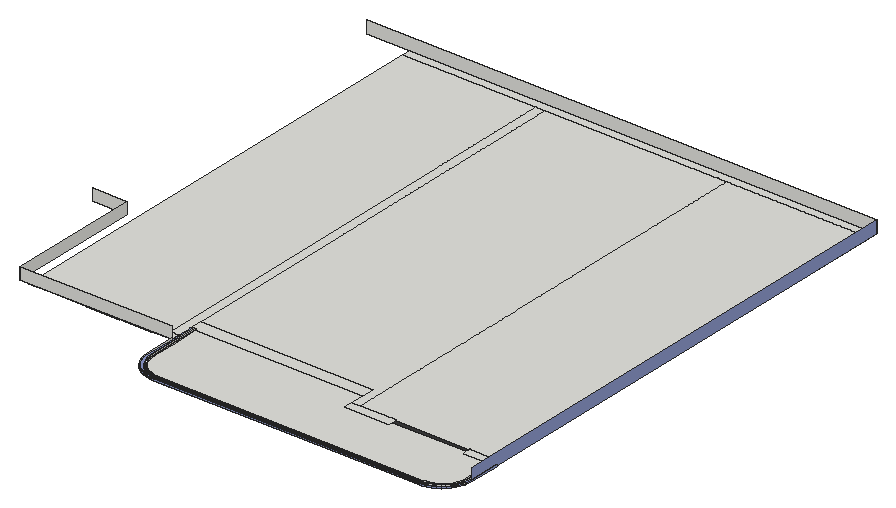
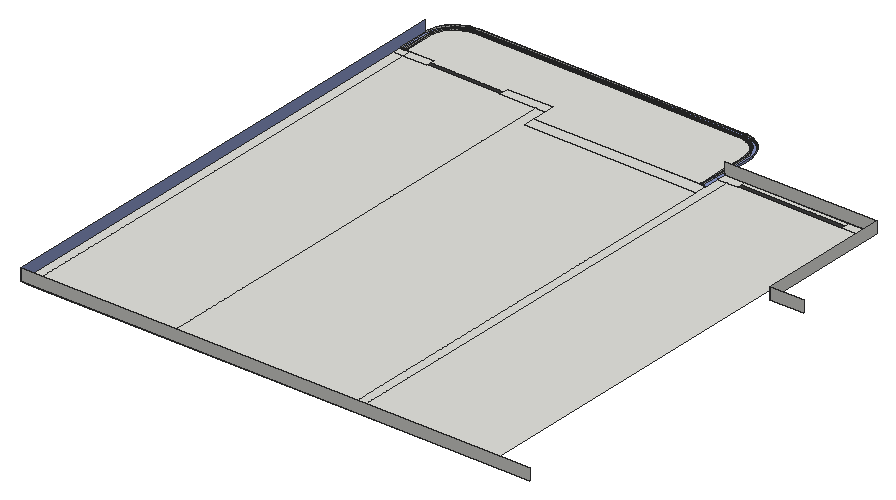
# SketchUp Ruby script. Lengths in inches.
U = 1.inch
M = Sketchup.active_model
def pt(a) = Geom::Point3d.new(a.map { |v| v * U })
def face(e, loops, mat)
  f = e.add_face(loops[0].map { |a| pt(a) })
  loops[1..].each { |l| e.add_face(l.map { |a| pt(a) }).erase! }
  f.material = f.back_material = mat if mat
  f
end
# faces: each face lists its corners as indices into pts; further lists are holes
def faces(e, pts, list, mat = nil) = list.each { |f| face(e, (f[0].is_a?(Array) ? f : [f]).map { |l| l.map { |i| pts[i] } }, mat) }
# xy, xz, yz: faces in a plane at the given z, y or x. An outline is a flat list of corners, or four numbers for a rectangle; further outlines are holes
def ring(l) = l.size == 4 ? [[l[0], l[1]], [l[2], l[1]], [l[2], l[3]], [l[0], l[3]]] : l.each_slice(2).to_a
def flat(e, list, mat, &to3) = list.each { |f| face(e, (f[0].is_a?(Array) ? f : [f]).map { |l| ring(l).map { |u, v| to3.(u, v) } }, mat) }
def xy(e, z, list, mat = nil) = flat(e, list, mat) { |x, y| [x, y, z] }
def xz(e, y, list, mat = nil) = flat(e, list, mat) { |x, z| [x, y, z] }
def yz(e, x, list, mat = nil) = flat(e, list, mat) { |y, z| [x, y, z] }
def lines(e, pts, list) = list.each { |a, b| e.add_line(pt(pts[a]), pt(pts[b])) }
# prism: a flat outline (further loops are holes) pulled along v
def prism(e, loops, v, mat = nil)
  f = face(e, loops, mat); d = Geom::Vector3d.new(v.map { |x| x * U })
  f.pushpull(f.normal.samedirection?(d) ? d.length : -d.length)
end
def box(e, o, s, mat = nil) = prism(e, [[o, [o[0] + s[0], o[1], o[2]], [o[0] + s[0], o[1] + s[1], o[2]], [o[0], o[1] + s[1], o[2]]]], [0, 0, s[2]], mat)
def at(x, y, z, deg = 0) = Geom::Transformation.translation(pt([x, y, z])) * Geom::Transformation.rotation(ORIGIN, Z_AXIS, deg.degrees)
def axes(o, x, y, z) = Geom::Transformation.new([*x, 0, *y, 0, *z, 0, *pt(o).to_a, 1])
def part(name) = M.definitions.add(name)
# library, detail: a bought-in or finely detailed component or shape, given as its bounding box
def library(name, o, s) = part(name).tap { |d| box(d.entities, o, s) }
def detail(e, o, s) = box(e.add_group.entities, o, s)
def put(e, d, t, mat = nil) = e.add_instance(d, t).tap { |i| i.material = mat if mat }
def group(e, t, mat = nil) = e.add_group.tap { |g| g.transformation = t; g.material = mat if mat }.entities
root = M.entities
M.materials.add("0326 AP 7207 CLASSIC PURPLE").color = [140, 152, 201]
M.materials.add("[Color M07]").color = [58, 58, 58]
xy(root,116.35,[[69.16,90.75,96.8,92.5625],[100.57,90.75,134.3,92.5625],[137.83,90.75,166.03,92.5625]],"[Color M07]")
xy(root,116.87,[[412.91,90.75,441.92,92.125],[446.86,90.75,480.82,92.125]],"[Color M07]")
xy(root,120,[[220.41,29.57,216.92,29.79,213.5,30.47,210.2,31.6,207.06,33.14,204.16,35.08,201.54,37.38,199.24,40.01,197.3,42.91,195.75,46.04,194.63,49.34,193.95,52.77,193.72,56.25,193.72,109.85,194.29,109.85,194.29,56.25,194.52,52.84,195.18,49.49,196.28,46.26,197.79,43.19,199.69,40.35,201.94,37.79,204.51,35.53,207.35,33.64,210.41,32.125,213.65,31.03,217,30.36,220.41,30.14,487.28,30.14,490.8125,30.37,494.16,31.03,497.4,32.13,500.46,33.64,503.3,35.54,505.84,37.77,505.87,37.79,508.12,40.36,510.01,43.2,511.52,46.26,512.62,49.49,513.29,52.84,513.52,56.38,513.52,86.25,514.09,86.25,514.09,56.36,513.86,52.77,513.18,49.35,512.05,46.04,510.51,42.91,508.57,40.01,506.27,37.39,506.22,37.34,503.65,35.09,500.75,33.15,497.62,31.6,494.3125,30.48,490.89,29.8,487.3,29.57],[220.41,31.87,217.22,32.07,214.1,32.7,211.08,33.72,208.21,35.13,205.5625,36.9,203.16,39.01,201.0625,41.41,199.29,44.06,197.88,46.92,196.85,49.9375,196.23,53.07,196.02,56.25,196.02,109.85,364.41,109.85,364.41,86.25,409.78,86.25,409.78,90.75,483.95,90.75,483.95,86.25,511.79,86.25,511.79,56.43,511.57,53.07,510.95,49.94,509.92,46.92,508.51,44.0625,506.74,41.41,504.64,39.02,502.24,36.91,499.59,35.14,496.73,33.73,493.71,32.71,490.59,32.09,487.22,31.87],[46.41,86.25,65.51,95.25],[65.51,86.25,169.68,90.75],[169.68,86.25,189.84,95.25],
  [189.84,86.25,190.41,95.25],[364.41,86.25,409.78,95.25],[483.95,86.25,508.41,95.25],[508.41,86.25,513.52,86.25,513.52,86.82,517.41,86.82,517.41,95.25,508.41,95.25],[513.52,86.25,517.41,86.82],
  [65.51,94.4375,65.51,95.25,46.41,95.25,46.41,557.25,181.41,557.25,181.41,95.25,169.68,95.25,169.68,94.4375],[409.78,94.5625,409.78,95.25,373.41,95.25,373.41,557.25,508.41,557.25,508.41,95.25,483.95,95.25,483.95,94.5625],[181.41,95.25,181.41,557.25,190.41,557.25,190.41,110.42,189.84,110.42,189.84,95.25],[189.84,95.25,190.41,110.42],[364.41,95.25,364.41,122.61,190.41,122.61,190.41,557.25,373.41,557.25,373.41,95.25],
  [364.41,95.25,373.41,557.25],[508.41,95.25,517.41,566.25],[190.41,109.85,194.29,110.42],[194.29,109.85,194.29,110.42,190.41,110.42,190.41,122.61,364.41,122.61,364.41,109.85],[46.41,557.25,508.41,566.25]])
xy(root,120,[[220.41,25.68,216.42,25.94,212.49,26.72,208.71,28.01,205.12,29.77,201.8,32,198.79,34.63,196.15,37.64,193.93,40.96,192.16,44.55,190.88,48.34,190.1,52.26,189.84,56.25,189.84,86.25,190.41,86.25,190.41,56.25,190.66,52.33,191.43,48.49,192.69,44.77,194.43,41.25,196.61,37.99,199.19,35.04,202.14,32.45,205.41,30.27,208.93,28.53,212.64,27.27,216.49,26.51,220.41,26.25,487.41,26.25,491.32,26.51,495.17,27.27,498.89,28.53,502.41,30.27,505.67,32.45,508.41,34.85,508.62,35.04,511.21,37.99,513.39,41.25,515.125,44.77,516.38,48.49,517.15,52.33,517.41,56.25,517.41,86.82,517.98,86.82,517.98,56.23,517.72,52.26,516.9375,48.34,515.65,44.55,513.88,40.96,511.66,37.64,509.02,34.63,508.78,34.42,506.02,32,502.69,29.77,499.11,28,495.32,26.72,491.4,25.9375,487.43,25.68],[220.41,26.25,216.49,26.51,212.64,27.27,208.93,28.53,205.41,30.27,202.14,32.45,199.19,35.04,196.61,37.99,194.43,41.25,192.69,44.77,191.43,48.49,190.66,52.33,190.41,56.25,190.41,109.85,193.72,109.85,193.72,56.25,193.95,52.77,194.63,49.34,195.75,46.04,197.3,42.91,199.24,40.01,201.54,37.38,204.16,35.08,207.06,33.14,210.2,31.6,213.5,30.47,216.92,29.79,220.41,29.57,487.3,29.57,490.89,29.8,494.3125,30.48,497.62,31.6,500.75,33.15,503.65,35.09,506.22,37.34,506.27,37.39,508.57,40.01,510.51,42.91,512.05,46.04,513.18,49.35,513.86,52.77,514.09,56.36,514.09,86.25,517.41,86.25,517.41,56.25,517.15,52.33,516.38,48.49,515.125,44.77,513.39,41.25,511.21,37.99,508.62,35.04,508.41,34.85,505.67,32.45,502.41,30.27,498.89,28.53,495.17,27.27,491.32,26.51,487.41,26.25]],"0326 AP 7207 CLASSIC PURPLE")
xy(root,120,[[65.51,90.75,169.68,94.4375],[409.78,90.75,483.95,94.5625]],"[Color M07]")
xz(root,25.68,[[220.41,120,487.43,121.1875]],"0326 AP 7207 CLASSIC PURPLE")
xz(root,26.25,[[220.41,120,487.41,121.1875]])
xz(root,29.57,[[220.41,120,487.3,120.9375]])
xz(root,30.14,[[220.41,120,487.28,120.625]])
xz(root,31.87,[[220.41,120,487.22,120.625]])
xz(root,86.25,[[37.41,120,189.84,120,189.84,121.1875,190.41,121.1875,190.41,132,37.41,132],[189.84,120,190.41,121.1875],[511.79,120,513.52,120.625],[513.52,120,514.09,120,514.09,120.9375,511.79,120.9375,511.79,120.625,513.52,120.625]])
xz(root,86.82,[[517.41,120,517.98,121.1875]])
xz(root,109.85,[[193.72,120,194.29,120,194.29,120.625,196.02,120.625,196.02,120.9375,193.72,120.9375],[194.29,120,196.02,120.625]])
xz(root,220.92,[[2.97,120,37.41,132]])
xz(root,566.25,[[2.97,120,517.41,132]])
yz(root,37.41,[[86.25,120,220.92,132]])
yz(root,189.84,[[56.25,120,86.25,121.1875]],"0326 AP 7207 CLASSIC PURPLE")
yz(root,190.41,[[56.25,120,86.25,121.1875]])
yz(root,193.72,[[56.25,120,86.25,120.9375],[86.25,120,95.25,120.9375],[95.25,120,109.85,120.9375]])
yz(root,194.29,[[56.25,120,86.25,120.625],[86.25,120,95.25,120.625],[95.25,120,109.85,120.625]])
yz(root,196.02,[[56.25,120,86.25,120.625],[86.25,120,109.85,120.625]])
yz(root,511.79,[[56.43,120,86.25,120.625]])
yz(root,513.52,[[56.38,120,86.25,120.625]])
yz(root,514.09,[[56.36,120,86.25,120.9375]])
yz(root,517.41,[[56.25,120,86.25,121.1875],[86.25,120,86.82,121.1875]])
yz(root,517.41,[[86.82,120,566.25,120,566.25,132,86.25,132,86.25,132.125,56.25,132.125,56.25,121.1875,86.82,121.1875]],"0326 AP 7207 CLASSIC PURPLE")
yz(root,517.98,[[56.23,120,86.82,121.1875]],"0326 AP 7207 CLASSIC PURPLE")
p = [[249.8,113.47,100.45],[250.52,113.47,101.11],[250.52,112.66,101.11],[249.8,112.66,100.45],[255.92,113.47,100.37],[256.63,113.47,100.88],
  [256.63,112.66,100.88],[255.92,112.66,100.37],[297.92,113.47,100.88],[298.63,113.47,100.37],[298.63,112.66,100.37],[297.92,112.66,100.88],
  [304.03,113.47,101.11],[304.75,113.47,100.45],[304.75,112.66,100.45],[304.03,112.66,101.11],[250.52,122.61,101.11],[249.8,122.61,100.45],
  [304.75,122.61,100.45],[304.03,122.61,101.11],[240.98,109.85,101.42],[240.26,109.85,100.52],[240.26,112.66,100.52],[240.98,112.66,101.42],
  [314.3,109.85,100.52],[313.57,109.85,101.42],[313.57,112.66,101.42],[314.3,112.66,100.52],[257.36,113.47,101.38],[257.36,112.66,101.38],
  [297.19,113.47,101.38],[297.19,112.66,101.38],[251.25,113.47,101.76],[251.25,112.66,101.76],[303.3,113.47,101.76],[303.3,112.66,101.76],
  [251.25,122.61,101.76],[303.3,122.61,101.76],[241.72,109.85,102.3],[241.72,112.66,102.3],[312.83,109.85,102.3],[312.83,112.66,102.3],
  [258.1,113.47,101.86],[258.1,112.66,101.86],[296.45,113.47,101.86],[296.45,112.66,101.86],[252,113.47,102.38],[252,112.66,102.38],
  [302.55,113.47,102.38],[302.55,112.66,102.38],[252,122.61,102.38],[302.55,122.61,102.38],[258.85,113.47,102.32],[258.85,112.66,102.32],
  [295.7,113.47,102.32],[295.7,112.66,102.32],[242.49,109.85,103.16],[242.49,112.66,103.16],[312.0625,109.85,103.16],[312.0625,112.66,103.16],
  [259.61,113.47,102.76],[259.61,112.66,102.76],[294.94,113.47,102.76],[294.94,112.66,102.76],[252.77,113.47,102.99],[252.77,112.66,102.99],
  [301.78,113.47,102.99],[301.78,112.66,102.99],[252.77,122.61,102.99],[301.78,122.61,102.99],[260.38,113.47,103.18],[260.38,112.66,103.18],
  [294.17,113.47,103.18],[294.17,112.66,103.18],[253.55,113.47,103.58],[253.55,112.66,103.58],[301,113.47,103.58],[301,112.66,103.58],
  [253.55,122.61,103.58],[301,122.61,103.58],[243.27,109.85,104],[243.27,112.66,104],[311.28,109.85,104],[311.28,112.66,104],
  [261.16,113.47,103.58],[261.16,112.66,103.58],[293.39,113.47,103.58],[293.39,112.66,103.58],[254.34,113.47,104.15],[254.34,112.66,104.15],
  [261.95,113.47,103.97],[261.95,112.66,103.97],[292.6,113.47,103.97],[292.6,112.66,103.97],[300.21,113.47,104.15],[300.21,112.66,104.15],
  [254.34,122.61,104.15],[300.21,122.61,104.15],[244.08,109.85,104.82],[244.08,112.66,104.82],[310.47,109.85,104.82],[310.47,112.66,104.82],
  [262.75,113.47,104.33],[262.75,112.66,104.33],[291.8,113.47,104.33],[291.8,112.66,104.33],[255.15,113.47,104.71],[255.15,112.66,104.71],
  [299.4,113.47,104.71],[299.4,112.66,104.71],[255.15,122.61,104.71],[299.4,122.61,104.71],[263.5625,113.47,104.68],[263.5625,112.66,104.68],
  [290.99,113.47,104.68],[290.99,112.66,104.68],[255.97,113.47,105.24],[255.97,112.66,105.24],[264.38,113.47,105],[264.38,112.66,105],
  [290.17,113.47,105],[290.17,112.66,105],[298.58,113.47,105.24],[298.58,112.66,105.24],[255.97,122.61,105.24],[298.58,122.61,105.24],
  [244.91,109.85,105.62],[244.91,112.66,105.62],[309.65,109.85,105.62],[309.65,112.66,105.62],[265.2,113.47,105.31],[265.2,112.66,105.31],
  [289.35,113.47,105.31],[289.35,112.66,105.31],[256.8,113.47,105.75],[256.8,112.66,105.75],[297.75,113.47,105.75],[297.75,112.66,105.75],
  [256.8,122.61,105.75],[297.75,122.61,105.75],[266.03,113.47,105.59],[266.03,112.66,105.59],[288.52,113.47,105.59],[288.52,112.66,105.59],
  [245.75,109.85,106.4],[245.75,112.66,106.4],[308.8,109.85,106.4],[308.8,112.66,106.4],[266.875,113.47,105.86],[266.875,112.66,105.86],
  [287.68,113.47,105.86],[287.68,112.66,105.86],[257.65,113.47,106.24],[257.65,112.66,106.24],[296.91,113.47,106.24],[296.91,112.66,106.24],
  [257.65,122.61,106.24],[296.91,122.61,106.24],[267.72,113.47,106.1],[267.72,112.66,106.1],[286.83,113.47,106.1],[286.83,112.66,106.1],
  [268.57,113.47,106.33],[268.57,112.66,106.33],[285.98,113.47,106.33],[285.98,112.66,106.33],[258.5,113.47,106.71],[258.5,112.66,106.71],
  [296.05,113.47,106.71],[296.05,112.66,106.71],[258.5,122.61,106.71],[296.05,122.61,106.71],[269.42,113.47,106.53],[269.42,112.66,106.53],
  [285.13,113.47,106.53],[285.13,112.66,106.53],[246.62,109.85,107.16],[246.62,112.66,107.16],[307.94,109.85,107.16],[307.94,112.66,107.16],
  [270.28,113.47,106.71],[270.28,112.66,106.71],[284.27,113.47,106.71],[284.27,112.66,106.71],[259.37,113.47,107.16],[259.37,112.66,107.16],
  [271.15,113.47,106.87],[271.15,112.66,106.87],[283.4,113.47,106.87],[283.4,112.66,106.87],[295.18,113.47,107.16],[295.18,112.66,107.16],
  [259.37,122.61,107.16],[295.18,122.61,107.16],[272.02,113.47,107.01],[272.02,112.66,107.01],[282.53,113.47,107.01],[282.53,112.66,107.01],
  [272.89,113.47,107.13],[272.89,112.66,107.13],[281.66,113.47,107.13],[281.66,112.66,107.13],[273.76,113.47,107.22],[273.76,112.66,107.22],
  [280.79,113.47,107.22],[280.79,112.66,107.22],[247.5,109.85,107.9],[247.5,112.66,107.9],[307.05,109.85,107.9],[307.05,112.66,107.9],
  [260.25,113.47,107.58],[260.25,112.66,107.58],[274.64,113.47,107.3],[274.64,112.66,107.3],[279.91,113.47,107.3],[279.91,112.66,107.3],
  [294.3,113.47,107.58],[294.3,112.66,107.58],[260.25,122.61,107.58],[294.3,122.61,107.58],[275.52,113.47,107.35],[275.52,112.66,107.35],
  [279.03,113.47,107.35],[279.03,112.66,107.35],[276.4,113.47,107.39],[276.4,112.66,107.39],[277.28,113.47,107.4],[277.28,112.66,107.4],
  [278.16,113.47,107.39],[278.16,112.66,107.39],[261.14,113.47,107.99],[261.14,112.66,107.99],[293.41,113.47,107.99],[293.41,112.66,107.99],
  [261.14,122.61,107.99],[293.41,122.61,107.99],[248.4,109.85,108.62],[248.4,112.66,108.62],[306.15,109.85,108.62],[306.15,112.66,108.62],
  [262.04,113.47,108.37],[262.04,112.66,108.37],[292.51,113.47,108.37],[292.51,112.66,108.37],[262.04,122.61,108.37],[292.51,122.61,108.37],
  [262.94,113.47,108.73],[262.94,112.66,108.73],[291.61,113.47,108.73],[291.61,112.66,108.73],[262.94,122.61,108.73],[291.61,122.61,108.73],
  [249.32,109.85,109.3125],[249.32,112.66,109.3125],[305.23,109.85,109.3125],[305.23,112.66,109.3125],[263.86,113.47,109.07],[263.86,112.66,109.07],
  [290.69,113.47,109.07],[290.69,112.66,109.07],[263.86,122.61,109.07],[290.69,122.61,109.07],[264.79,113.47,109.39],[264.79,112.66,109.39],
  [289.77,113.47,109.39],[289.77,112.66,109.39],[264.79,122.61,109.39],[289.77,122.61,109.39],[250.25,109.85,109.99],[250.25,112.66,109.99],
  [304.3,109.85,109.99],[304.3,112.66,109.99],[265.72,113.47,109.68],[265.72,112.66,109.68],[288.83,113.47,109.68],[288.83,112.66,109.68],
  [265.72,122.61,109.68],[288.83,122.61,109.68],[266.66,113.47,109.95],[266.66,112.66,109.95],[287.9,113.47,109.95],[287.9,112.66,109.95],
  [266.66,122.61,109.95],[287.9,122.61,109.95],[251.2,109.85,110.64],[251.2,112.66,110.64],[303.35,109.85,110.64],[303.35,112.66,110.64],
  [267.6,113.47,110.2],[267.6,112.66,110.2],[286.95,113.47,110.2],[286.95,112.66,110.2],[267.6,122.61,110.2],[286.95,122.61,110.2],
  [268.55,113.47,110.43],[268.55,112.66,110.43],[286,113.47,110.43],[286,112.66,110.43],[268.55,122.61,110.43],[286,122.61,110.43],
  [269.51,113.47,110.63],[269.51,112.66,110.63],[285.04,113.47,110.63],[285.04,112.66,110.63],[269.51,122.61,110.63],[285.04,122.61,110.63],
  [252.17,109.85,111.26],[252.17,112.66,111.26],[302.38,109.85,111.26],[302.38,112.66,111.26],[270.47,113.47,110.81],[270.47,112.66,110.81],
  [284.08,113.47,110.81],[284.08,112.66,110.81],[270.47,122.61,110.81],[284.08,122.61,110.81],[271.43,113.47,110.96],[271.43,112.66,110.96],
  [283.12,113.47,110.96],[283.12,112.66,110.96],[271.43,122.61,110.96],[283.12,122.61,110.96],[272.4,113.47,111.09],[272.4,112.66,111.09],
  [282.15,113.47,111.09],[282.15,112.66,111.09],[272.4,122.61,111.09],[282.15,122.61,111.09],[273.375,113.47,111.2],[273.375,112.66,111.2],
  [281.18,113.47,111.2],[281.18,112.66,111.2],[273.375,122.61,111.2],[281.18,122.61,111.2],[274.35,113.47,111.28],[274.35,112.66,111.28],
  [280.2,113.47,111.28],[280.2,112.66,111.28],[274.35,122.61,111.28],[280.2,122.61,111.28],[253.15,109.85,111.86],[253.15,112.66,111.86],
  [301.4,109.85,111.86],[301.4,112.66,111.86],[275.32,113.47,111.34],[275.32,112.66,111.34],[276.3,113.47,111.38],[276.3,112.66,111.38],
  [278.25,113.47,111.38],[279.23,113.47,111.34],[279.23,112.66,111.34],[278.25,112.66,111.38],[275.32,122.61,111.34],[276.3,122.61,111.38],
  [279.23,122.61,111.34],[278.25,122.61,111.38],[277.28,113.47,111.39],[277.28,112.66,111.39],[277.28,122.61,111.39],[254.15,109.85,112.44],
  [254.15,112.66,112.44],[300.41,109.85,112.44],[300.41,112.66,112.44],[255.16,109.85,112.99],[255.16,112.66,112.99],[299.4,109.85,112.99],
  [299.4,112.66,112.99],[256.18,109.85,113.52],[256.18,112.66,113.52],[298.37,109.85,113.52],[298.37,112.66,113.52],[257.21,109.85,114.03],
  [257.21,112.66,114.03],[297.34,109.85,114.03],[297.34,112.66,114.03],[258.26,109.85,114.5],[258.26,112.66,114.5],[296.29,109.85,114.5],
  [296.29,112.66,114.5],[259.32,109.85,114.96],[259.32,112.66,114.96],[295.23,109.85,114.96],[295.23,112.66,114.96],[260.39,109.85,115.38],
  [260.39,112.66,115.38],[294.16,109.85,115.38],[294.16,112.66,115.38],[261.47,109.85,115.78],[261.47,112.66,115.78],[293.08,109.85,115.78],
  [293.08,112.66,115.78],[262.56,109.85,116.15],[262.56,112.66,116.15],[291.99,109.85,116.15],[291.99,112.66,116.15],[263.66,109.85,116.5],
  [263.66,112.66,116.5],[290.89,109.85,116.5],[290.89,112.66,116.5],[264.76,109.85,116.82],[264.76,112.66,116.82],[289.79,109.85,116.82],
  [289.79,112.66,116.82],[265.88,109.85,117.11],[265.88,112.66,117.11],[288.67,109.85,117.11],[288.67,112.66,117.11],[267,109.85,117.38],
  [267,112.66,117.38],[287.55,109.85,117.38],[287.55,112.66,117.38],[268.125,109.85,117.62],[268.125,112.66,117.62],[286.43,109.85,117.62],
  [286.43,112.66,117.62],[269.26,109.85,117.83],[269.26,112.66,117.83],[285.3,109.85,117.83],[285.3,112.66,117.83],[270.39,109.85,118.01],
  [270.39,112.66,118.01],[284.16,109.85,118.01],[284.16,112.66,118.01],[271.53,109.85,118.16],[271.53,112.66,118.16],[283.02,109.85,118.16],
  [283.02,112.66,118.16],[272.68,109.85,118.29],[272.68,112.66,118.29],[281.875,109.85,118.29],[281.875,112.66,118.29],[273.83,109.85,118.39],
  [273.83,112.66,118.39],[280.73,109.85,118.39],[280.73,112.66,118.39],[274.97,109.85,118.46],[274.97,112.66,118.46],[279.58,109.85,118.46],
  [279.58,112.66,118.46],[276.125,109.85,118.5],[276.125,112.66,118.5],[277.28,109.85,118.51],[277.28,112.66,118.51],[278.43,109.85,118.5],
  [278.43,112.66,118.5],[216.42,25.94,120],[220.41,25.68,120],[220.41,25.68,121.1875],[216.42,25.94,121.1875],[487.43,25.68,120],
  [491.4,25.9375,120],[491.4,25.9375,121.1875],[487.43,25.68,121.1875],[212.49,26.72,120],[212.49,26.72,121.1875],[495.32,26.72,120],
  [495.32,26.72,121.1875],[220.41,26.25,120],[220.41,26.25,121.1875],[216.49,26.51,121.1875],[216.49,26.51,120],[491.32,26.51,120],
  [491.32,26.51,121.1875],[487.41,26.25,121.1875],[487.41,26.25,120],[212.64,27.27,121.1875],[212.64,27.27,120],[495.17,27.27,120],
  [495.17,27.27,121.1875],[208.71,28.01,120],[208.71,28.01,121.1875],[499.11,28,120],[499.11,28,121.1875],[208.93,28.53,121.1875],
  [208.93,28.53,120],[498.89,28.53,120],[498.89,28.53,121.1875],[205.12,29.77,120],[205.12,29.77,121.1875],[502.69,29.77,120],
  [502.69,29.77,121.1875],[205.41,30.27,121.1875],[205.41,30.27,120],[502.41,30.27,120],[502.41,30.27,121.1875],[220.41,29.57,120],
  [216.92,29.79,120],[216.92,29.79,120.9375],[220.41,29.57,120.9375],[490.89,29.8,120],[487.3,29.57,120],[487.3,29.57,120.9375],
  [490.89,29.8,120.9375],[201.8,32,120],[201.8,32,121.1875],[213.5,30.47,120],[213.5,30.47,120.9375],[494.3125,30.48,120],
  [494.3125,30.48,120.9375],[506.02,32,120],[506.02,32,121.1875],[220.41,30.14,120],[217,30.36,120],[217,30.36,120.625],
  [220.41,30.14,120.625],[490.8125,30.37,120],[487.28,30.14,120],[487.28,30.14,120.625],[490.8125,30.37,120.625],[202.14,32.45,121.1875],
  [202.14,32.45,120],[505.67,32.45,120],[505.67,32.45,121.1875],[213.65,31.03,120],[213.65,31.03,120.625],[494.16,31.03,120],
  [494.16,31.03,120.625],[210.2,31.6,120],[210.2,31.6,120.9375],[497.62,31.6,120],[497.62,31.6,120.9375],[210.41,32.125,120],
  [210.41,32.125,120.625],[497.4,32.13,120],[497.4,32.13,120.625],[207.06,33.14,120],[207.06,33.14,120.9375],[500.75,33.15,120],
  [500.75,33.15,120.9375],[217.22,32.07,120],[220.41,31.87,120],[220.41,31.87,120.625],[217.22,32.07,120.625],[487.22,31.87,120],
  [490.59,32.09,120],[490.59,32.09,120.625],[487.22,31.87,120.625],[198.79,34.63,120],[198.79,34.63,121.1875],[508.78,34.42,120],
  [508.78,34.42,121.1875],[207.35,33.64,120],[207.35,33.64,120.625],[214.1,32.7,120],[214.1,32.7,120.625],[493.71,32.71,120],
  [493.71,32.71,120.625],[500.46,33.64,120],[500.46,33.64,120.625],[199.19,35.04,121.1875],[199.19,35.04,120],[508.41,34.85,120],
  [508.41,34.85,121.1875],[211.08,33.72,120],[211.08,33.72,120.625],[496.73,33.73,120],[496.73,33.73,120.625],[204.16,35.08,120],
  [204.16,35.08,120.9375],[503.65,35.09,120],[503.65,35.09,120.9375],[204.51,35.53,120],[204.51,35.53,120.625],[503.3,35.54,120],
  [503.3,35.54,120.625],[208.21,35.13,120],[208.21,35.13,120.625],[499.59,35.14,120],[499.59,35.14,120.625],[509.02,34.63,120],
  [509.02,34.63,121.1875],[196.15,37.64,120],[196.15,37.64,121.1875],[511.66,37.64,120],[511.66,37.64,121.1875],[508.62,35.04,120],
  [508.62,35.04,121.1875],[196.61,37.99,121.1875],[196.61,37.99,120],[511.21,37.99,120],[511.21,37.99,121.1875],[201.54,37.38,120],
  [201.54,37.38,120.9375],[205.5625,36.9,120],[205.5625,36.9,120.625],[502.24,36.91,120],[502.24,36.91,120.625],[506.22,37.34,120],
  [506.22,37.34,120.9375],[201.94,37.79,120],[201.94,37.79,120.625],[505.84,37.77,120],[505.84,37.77,120.625],[203.16,39.01,120],
  [203.16,39.01,120.625],[504.64,39.02,120],[504.64,39.02,120.625],[506.27,37.39,120],[506.27,37.39,120.9375],[199.24,40.01,120],
  [199.24,40.01,120.9375],[508.57,40.01,120],[508.57,40.01,120.9375],[193.93,40.96,120],[193.93,40.96,121.1875],[513.88,40.96,120],
  [513.88,40.96,121.1875],[199.69,40.35,120],[199.69,40.35,120.625],[505.87,37.79,120],[505.87,37.79,120.625],[508.12,40.36,120],
  [508.12,40.36,120.625],[194.43,41.25,121.1875],[194.43,41.25,120],[513.39,41.25,120],[513.39,41.25,121.1875],[201.0625,41.41,120],
  [201.0625,41.41,120.625],[506.74,41.41,120],[506.74,41.41,120.625],[197.3,42.91,120],[197.3,42.91,120.9375],[510.51,42.91,120],
  [510.51,42.91,120.9375],[197.79,43.19,120],[197.79,43.19,120.625],[510.01,43.2,120],[510.01,43.2,120.625],[192.16,44.55,120],
  [192.16,44.55,121.1875],[515.65,44.55,120],[515.65,44.55,121.1875],[192.69,44.77,121.1875],[192.69,44.77,120],[515.125,44.77,120],
  [515.125,44.77,121.1875],[199.29,44.06,120],[199.29,44.06,120.625],[508.51,44.0625,120],[508.51,44.0625,120.625],[195.75,46.04,120],
  [195.75,46.04,120.9375],[512.05,46.04,120],[512.05,46.04,120.9375],[196.28,46.26,120],[196.28,46.26,120.625],[511.52,46.26,120],
  [511.52,46.26,120.625],[197.88,46.92,120],[197.88,46.92,120.625],[509.92,46.92,120],[509.92,46.92,120.625],[190.88,48.34,120],
  [190.88,48.34,121.1875],[516.9375,48.34,120],[516.9375,48.34,121.1875],[191.43,48.49,121.1875],[191.43,48.49,120],[516.38,48.49,120],
  [516.38,48.49,121.1875],[194.63,49.34,120],[194.63,49.34,120.9375],[513.18,49.35,120],[513.18,49.35,120.9375],[195.18,49.49,120],
  [195.18,49.49,120.625],[512.62,49.49,120],[512.62,49.49,120.625],[196.85,49.9375,120],[196.85,49.9375,120.625],[510.95,49.94,120],
  [510.95,49.94,120.625],[190.1,52.26,120],[190.1,52.26,121.1875],[517.72,52.26,120],[517.72,52.26,121.1875],[190.66,52.33,121.1875],
  [190.66,52.33,120],[517.15,52.33,120],[517.15,52.33,121.1875],[193.95,52.77,120],[193.95,52.77,120.9375],[513.86,52.77,120],
  [513.86,52.77,120.9375],[194.52,52.84,120],[194.52,52.84,120.625],[513.29,52.84,120],[513.29,52.84,120.625],[196.23,53.07,120],
  [196.23,53.07,120.625],[511.57,53.07,120],[511.57,53.07,120.625],[189.84,56.25,120],[189.84,56.25,121.1875],[190.41,56.25,121.1875],
  [190.41,56.25,120],[517.41,56.25,120],[517.41,56.25,121.1875],[517.98,56.23,120],[517.98,56.23,121.1875],[193.72,56.25,120],
  [193.72,56.25,120.9375],[194.29,56.25,120],[194.29,56.25,120.625],[513.52,56.38,120],[513.52,56.38,120.625],[514.09,56.36,120],
  [514.09,56.36,120.9375],[196.02,56.25,120],[196.02,56.25,120.625],[511.79,56.43,120],[511.79,56.43,120.625]]
faces(root,p,[[0,1,2,3],[4,5,6,7],[8,9,10,11],[12,13,14,15],[5,28,29,6],[30,8,11,31],[1,32,33,2],[34,12,15,35],
  [28,42,43,29],[44,30,31,45],[32,46,47,33],[48,34,35,49],[42,52,53,43],[54,44,45,55],[52,60,61,53],[62,54,55,63],
  [46,64,65,47],[66,48,49,67],[60,70,71,61],[72,62,63,73],[64,74,75,65],[76,66,67,77],[70,84,85,71],[86,72,73,87],
  [74,88,89,75],[84,90,91,85],[92,86,87,93],[94,76,77,95],[90,102,103,91],[104,92,93,105],[88,106,107,89],[108,94,95,109],
  [102,112,113,103],[114,104,105,115],[106,116,117,107],[112,118,119,113],[120,114,115,121],[122,108,109,123],[118,130,131,119],[132,120,121,133],
  [116,134,135,117],[136,122,123,137],[130,140,141,131],[142,132,133,143],[140,148,149,141],[150,142,143,151],[134,152,153,135],[154,136,137,155],
  [148,158,159,149],[160,150,151,161],[158,162,163,159],[164,160,161,165],[152,166,167,153],[168,154,155,169],[162,172,173,163],[174,164,165,175],
  [172,180,181,173],[182,174,175,183],[166,184,185,167],[180,186,187,181],[188,182,183,189],[190,168,169,191],[186,194,195,187],[196,188,189,197],
  [194,198,199,195],[200,196,197,201],[198,202,203,199],[204,200,201,205],[184,210,211,185],[202,212,213,203],[214,204,205,215],[216,190,191,217],
  [212,220,221,213],[222,214,215,223],[220,224,225,221],[224,226,227,225],[226,228,229,227],[228,222,223,229],[210,230,231,211],[232,216,217,233],
  [230,240,241,231],[242,232,233,243],[240,246,247,241],[248,242,243,249],[246,256,257,247],[258,248,249,259],[256,262,263,257],[264,258,259,265],
  [262,272,273,263],[274,264,265,275],[272,278,279,273],[280,274,275,281],[278,288,289,279],[290,280,281,291],[288,294,295,289],[296,290,291,297],
  [294,300,301,295],[302,296,297,303],[300,310,311,301],[312,302,303,313],[310,316,317,311],[318,312,313,319],[316,322,323,317],[324,318,319,325],
  [322,328,329,323],[330,324,325,331],[328,334,335,329],[336,330,331,337],[334,344,345,335],[344,346,347,345],[348,349,350,351],[349,336,337,350],
  [346,356,357,347],[356,348,351,357]],"[Color M07]")
faces(root,p,[[16,1,0,17],[18,13,12,19],[20,21,22,23],[24,25,26,27],[36,32,1,16],[19,12,34,37],[38,20,23,39],[25,40,41,26],
  [50,46,32,36],[37,34,48,51],[56,38,39,57],[40,58,59,41],[68,64,46,50],[51,48,66,69],[78,74,64,68],[69,66,76,79],
  [80,56,57,81],[58,82,83,59],[96,88,74,78],[79,76,94,97],[98,80,81,99],[82,100,101,83],[110,106,88,96],[97,94,108,111],
  [124,116,106,110],[111,108,122,125],[126,98,99,127],[100,128,129,101],[138,134,116,124],[125,122,136,139],[144,126,127,145],[128,146,147,129],
  [156,152,134,138],[139,136,154,157],[170,166,152,156],[157,154,168,171],[176,144,145,177],[146,178,179,147],[192,184,166,170],[171,168,190,193],
  [206,176,177,207],[178,208,209,179],[218,210,184,192],[193,190,216,219],[234,230,210,218],[219,216,232,235],[236,206,207,237],[208,238,239,209],
  [244,240,230,234],[235,232,242,245],[250,246,240,244],[245,242,248,251],[252,236,237,253],[238,254,255,239],[260,256,246,250],[251,248,258,261],
  [266,262,256,260],[261,258,264,267],[268,252,253,269],[254,270,271,255],[276,272,262,266],[267,264,274,277],[282,278,272,276],[277,274,280,283],
  [284,268,269,285],[270,286,287,271],[292,288,278,282],[283,280,290,293],[298,294,288,292],[293,290,296,299],[304,300,294,298],[299,296,302,305],
  [306,284,285,307],[286,308,309,287],[314,310,300,304],[305,302,312,315],[320,316,310,314],[315,312,318,321],[326,322,316,320],[321,318,324,327],
  [332,328,322,326],[327,324,330,333],[338,334,328,332],[333,330,336,339],[340,306,307,341],[308,342,343,309],[352,344,334,338],[353,346,344,352],
  [354,349,348,355],[339,336,349,354],[358,356,346,353],[355,348,356,358],[359,340,341,360],[342,361,362,343],[363,359,360,364],[361,365,366,362],
  [367,363,364,368],[365,369,370,366],[371,367,368,372],[369,373,374,370],[375,371,372,376],[373,377,378,374],[379,375,376,380],[377,381,382,378],
  [383,379,380,384],[381,385,386,382],[387,383,384,388],[385,389,390,386],[391,387,388,392],[389,393,394,390],[395,391,392,396],[393,397,398,394],
  [399,395,396,400],[397,401,402,398],[403,399,400,404],[401,405,406,402],[407,403,404,408],[405,409,410,406],[411,407,408,412],[409,413,414,410],
  [415,411,412,416],[413,417,418,414],[419,415,416,420],[417,421,422,418],[423,419,420,424],[421,425,426,422],[427,423,424,428],[425,429,430,426],
  [431,427,428,432],[429,433,434,430],[435,431,432,436],[433,437,438,434],[439,435,436,440],[441,439,440,442],[443,441,442,444],[437,443,444,438],
  [457,458,459,460],[461,462,463,464],[460,459,465,466],[467,468,462,461],[466,465,473,474],[475,476,468,467],[474,473,481,482],[483,484,476,475],
  [485,486,487,488],[489,490,491,492],[486,495,496,487],[497,489,492,498],[501,502,503,504],[505,506,507,508],[482,481,509,510],[511,512,484,483],
  [502,513,514,503],[515,505,508,516],[495,517,518,496],[519,497,498,520],[513,521,522,514],[523,515,516,524],[517,525,526,518],[527,519,520,528],
  [529,530,531,532],[533,534,535,536],[521,541,542,522],[543,529,532,544],[534,545,546,535],[547,523,524,548],[510,509,549,550],[511,551,552,512],
  [553,543,544,554],[545,555,556,546],[525,557,558,526],[559,527,528,560],[541,561,562,542],[563,547,548,564],[565,553,554,566],[555,567,568,556],
  [575,551,552,576],[550,549,577,578],[579,580,576,575],[557,581,582,558],[583,565,566,584],[567,585,586,568],[587,559,560,588],[561,589,590,562],
  [591,563,564,592],[593,583,584,594],[585,595,596,586],[597,587,588,598],[581,599,600,582],[601,597,598,602],[589,607,608,590],[609,591,592,610],
  [611,609,610,612],[578,577,613,614],[615,616,580,579],[617,593,594,618],[595,619,620,596],[599,621,622,600],[623,601,602,624],[607,625,626,608],
  [627,611,612,628],[614,613,633,634],[635,636,616,615],[637,617,618,638],[619,639,640,620],[621,641,642,622],[643,623,624,644],[625,645,646,626],
  [647,627,628,648],[649,637,638,650],[639,651,652,640],[634,633,657,658],[659,660,636,635],[641,661,662,642],[663,643,644,664],[645,665,666,646],
  [667,647,648,668],[669,649,650,670],[651,671,672,652],[658,657,677,678],[679,680,660,659],[661,681,682,662],[683,663,664,684],[665,685,686,666],
  [687,667,668,688],[689,669,670,690],[671,691,692,672],[678,677,695,696],[697,698,680,679],[681,701,702,682],[685,703,704,686],[705,687,688,706],
  [707,683,684,708],[709,689,690,710],[691,711,712,692]])
faces(root,p,[[445,446,447,448],[449,450,451,452],[453,445,448,454],[450,455,456,451],[469,453,454,470],[455,471,472,456],[477,469,470,478],[471,479,480,472],
  [493,477,478,494],[479,499,500,480],[537,493,494,538],[499,539,540,500],[539,569,570,540],[571,537,538,572],[569,573,574,570],[603,571,572,604],
  [573,605,606,574],[629,603,604,630],[605,631,632,606],[653,629,630,654],[631,655,656,632],[673,653,654,674],[655,675,676,656],[693,673,674,694],
  [675,699,700,676]],"0326 AP 7207 CLASSIC PURPLE")
